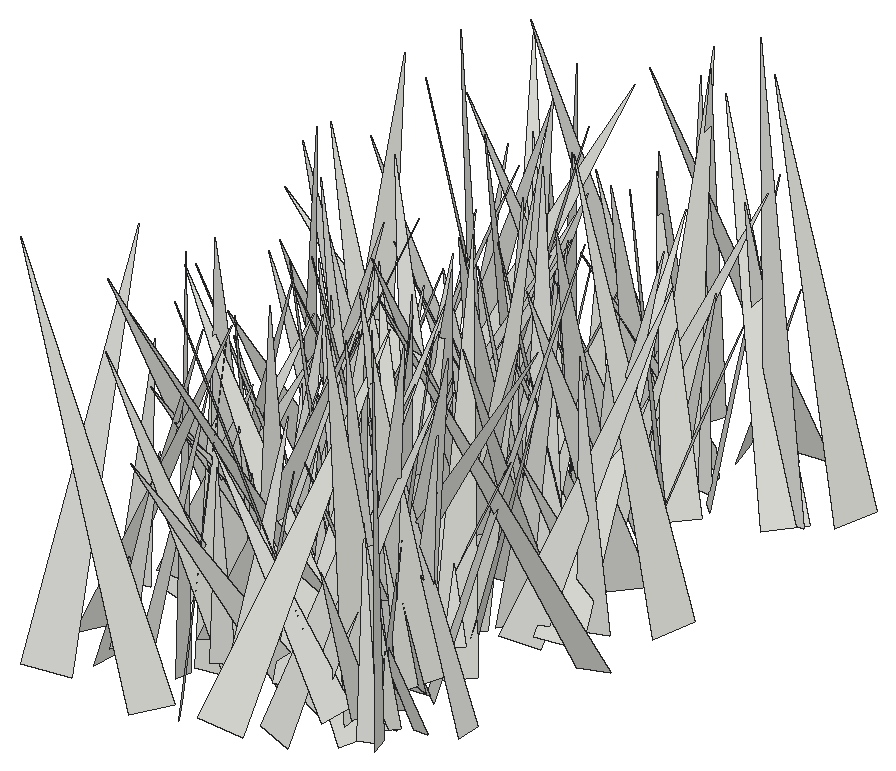
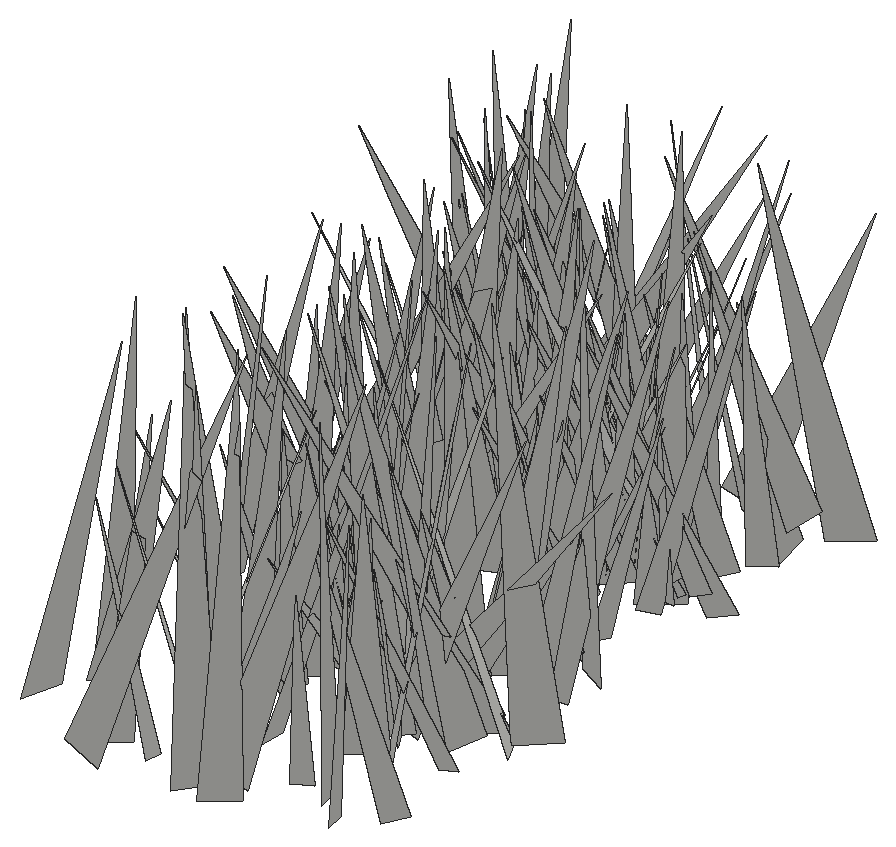
# SketchUp Ruby script. Lengths in inches.
U = 1.inch
M = Sketchup.active_model
def pt(a) = Geom::Point3d.new(a.map { |v| v * U })
def face(e, loops, mat)
  f = e.add_face(loops[0].map { |a| pt(a) })
  loops[1..].each { |l| e.add_face(l.map { |a| pt(a) }).erase! }
  f.material = f.back_material = mat if mat
  f
end
# faces: each face lists its corners as indices into pts; further lists are holes
def faces(e, pts, list, mat = nil) = list.each { |f| face(e, (f[0].is_a?(Array) ? f : [f]).map { |l| l.map { |i| pts[i] } }, mat) }
# xy, xz, yz: faces in a plane at the given z, y or x. An outline is a flat list of corners, or four numbers for a rectangle; further outlines are holes
def ring(l) = l.size == 4 ? [[l[0], l[1]], [l[2], l[1]], [l[2], l[3]], [l[0], l[3]]] : l.each_slice(2).to_a
def flat(e, list, mat, &to3) = list.each { |f| face(e, (f[0].is_a?(Array) ? f : [f]).map { |l| ring(l).map { |u, v| to3.(u, v) } }, mat) }
def xy(e, z, list, mat = nil) = flat(e, list, mat) { |x, y| [x, y, z] }
def xz(e, y, list, mat = nil) = flat(e, list, mat) { |x, z| [x, y, z] }
def yz(e, x, list, mat = nil) = flat(e, list, mat) { |y, z| [x, y, z] }
def lines(e, pts, list) = list.each { |a, b| e.add_line(pt(pts[a]), pt(pts[b])) }
# prism: a flat outline (further loops are holes) pulled along v
def prism(e, loops, v, mat = nil)
  f = face(e, loops, mat); d = Geom::Vector3d.new(v.map { |x| x * U })
  f.pushpull(f.normal.samedirection?(d) ? d.length : -d.length)
end
def box(e, o, s, mat = nil) = prism(e, [[o, [o[0] + s[0], o[1], o[2]], [o[0] + s[0], o[1] + s[1], o[2]], [o[0], o[1] + s[1], o[2]]]], [0, 0, s[2]], mat)
def at(x, y, z, deg = 0) = Geom::Transformation.translation(pt([x, y, z])) * Geom::Transformation.rotation(ORIGIN, Z_AXIS, deg.degrees)
def axes(o, x, y, z) = Geom::Transformation.new([*x, 0, *y, 0, *z, 0, *pt(o).to_a, 1])
def part(name) = M.definitions.add(name)
# library, detail: a bought-in or finely detailed component or shape, given as its bounding box
def library(name, o, s) = part(name).tap { |d| box(d.entities, o, s) }
def detail(e, o, s) = box(e.add_group.entities, o, s)
def put(e, d, t, mat = nil) = e.add_instance(d, t).tap { |i| i.material = mat if mat }
def group(e, t, mat = nil) = e.add_group.tap { |g| g.transformation = t; g.material = mat if mat }.entities
root = M.entities
c1 = part("fur_instance\#9")
p = [[0.8125,0,1.79],[0.67,-0.02,1.48],[0,-0.11,0],[0,0.11,0]]
faces(c1.entities,p,[[0,1,2,3]])
put(root,c1,axes([143.54,146.02,-28.22],[2.44843,-5.51273,0.60157],[-4.8536,-2.44839,-2.68234],[-2.6823,-0.60174,5.40279]))
put(root,c1,axes([140.68,143.08,-28.22],[5.52113,3.74347,2.2115],[4.00437,-5.77059,-0.2291],[-1.6939,-1.44011,6.66663]))
put(root,c1,axes([146.79,144.82,-27.1],[3.04717,-2.22298,0.43436],[-2.028,-3.00193,-1.13631],[-1.00873,-0.67996,3.59662]))
put(root,c1,axes([140.03,142.41,-28.22],[-2.68904,7.46116,1.26428],[7.06219,1.99214,3.26422],[-2.71897,-2.20471,7.22805]))
put(root,c1,axes([143.4375,143.2,-27.1],[4.00682,1.30969,1.18737],[1.29487,-4.17692,0.23764],[-1.20352,-0.13365,4.20874]))
put(root,c1,axes([146.1,144.29,-27.1],[-4.58905,2.11277,0.48874],[2.15665,4.32669,1.54618],[-0.22698,-1.60562,4.80963]))
put(root,c1,axes([138,143.41,-27.1],[3.18405,-1.52738,1.26596],[-1.78098,-3.25535,0.55182],[-0.87386,1.06936,3.48806]))
put(root,c1,axes([143.01,143.0625,-27.1],[-1.4542,4.67664,1.33998],[4.76533,1.65076,-0.58976],[0.97884,-1.08869,4.86188]))
put(root,c1,axes([135.78,142.31,-28.22],[-2.77927,7.20298,1.80131],[7.21654,3.07297,-1.15349],[1.74623,-1.2353,7.63392]))
put(root,c1,axes([145.125,145.05,-27.1],[-5.01465,-5.39389,0.78065],[-5.43536,4.87162,-1.25473],[-0.40033,1.42249,7.25716]))
put(root,c1,axes([143.71,141.3125,-27.1],[-2.62249,6.7547,0.84995],[6.3246,2.75431,-2.37468],[2.5195,0.11678,6.84575]))
put(root,c1,axes([141.24,145.7,-28.22],[-6.5147,0.26004,1.16019],[0.55336,6.38259,1.67669],[1.05235,-1.74639,6.3006]))
put(root,c1,axes([147.95,143.54,-27.1],[-0.46969,3.55211,0.73396],[3.59032,0.35011,0.60316],[-0.51554,-0.79795,3.53189]))
put(root,c1,axes([141.16,144.64,-27.1],[1.90593,-3.10212,1.28599],[-3.27722,-2.04084,-0.06594],[-0.73267,1.05893,3.64024]))
put(root,c1,axes([136.45,143.83,-27.1],[6.61677,-1.08212,0.53072],[-1.15649,-6.53431,1.0953],[-0.3394,1.16883,6.6146]))
put(root,c1,axes([146.45,145.71,-28.22],[4.88048,-6.02987,2.56967],[-6.14977,-5.32095,-0.80587],[-2.26779,1.4525,7.7155]))
put(root,c1,axes([138.1875,144.61,-27.1],[2.95558,3.83246,1.3061],[4.0436,-2.87668,-0.7093],[-0.20723,-1.47175,4.78749]))
put(root,c1,axes([148.43,143.57,-27.1],[-6.12572,-2.31991,2.2614],[-2.97153,5.95041,-1.94497],[1.2907,2.68904,6.25488]))
put(root,c1,axes([146.09,147.31,-28.22],[-2.23996,-8.03771,0.28468],[-7.44594,1.96073,-3.22749],[-3.04036,1.11981,7.69451]))
put(root,c1,axes([136.8125,144.06,-28.22],[6.05583,0.88682,1.38397],[0.67013,-6.15634,1.01257],[-1.50092,0.82941,6.03608]))
put(root,c1,axes([144.86,144.31,-27.1],[1.84734,5.85191,0.92453],[5.8229,-1.61485,-1.41361],[1.09242,-1.28828,5.97153]))
put(root,c1,axes([146.15,146.26,-28.22],[0.04247,-7.07988,2.41623],[-7.48051,-0.06275,-0.05238],[-0.06984,2.41579,7.07981]))
put(root,c1,axes([138.84,147.71,-27.1],[3.08843,-3.08617,0.55459],[-2.71507,-3.02147,-1.69397],[-1.56857,-0.84658,4.0241]))
put(root,c1,axes([140.03,145.85,-27.1],[6.60673,-3.01857,0.44503],[-3.04917,-6.49303,1.22551],[0.11127,1.29906,7.15953]))
put(root,c1,axes([141.49,146.93,-28.22],[6.66168,-2.88093,2.18206],[-2.80757,-7.00677,-0.67958],[-2.27567,0.211,7.22605]))
put(root,c1,axes([147.64,146.68,-28.22],[-2.3451,-4.39084,0.71964],[-4.31416,2.04482,-1.58228],[-1.08875,1.35503,4.71968]))
put(root,c1,axes([146.47,145.2,-28.22],[-4.02573,7.19257,0.41274],[6.48293,3.4104,3.80141],[-3.14246,-2.17854,7.31361]))
put(root,c1,axes([143.54,144.78,-27.1],[-0.09668,3.9627,0.07364],[3.92699,0.08582,0.53775],[-0.5359,-0.08606,3.92724]))
put(root,c1,axes([144.19,143.48,-28.22],[2.76635,7.35948,0.05567],[7.35952,-2.76581,-0.07342],[0.04914,-0.07794,7.86188]))
put(root,c1,axes([144.94,147.53,-28.22],[0.67729,-7.55263,2.0847],[-7.70125,-0.25666,1.57216],[1.44182,2.17688,7.41817]))
put(root,c1,axes([145.24,146.55,-27.1],[-2.81459,-5.30869,2.75415],[-5.79641,3.17103,0.18862],[1.47279,2.33491,6.00571]))
put(root,c1,axes([145.86,148.62,-28.22],[0.26999,-5.16111,0.17986],[-5.16087,-0.27616,-0.17741],[-0.18667,0.17024,5.16512]))
put(root,c1,axes([143.51,145.55,-27.1],[-1.89071,3.52857,0.74513],[3.44423,2.01617,-0.80816],[1.06925,-0.25501,3.92077]))
put(root,c1,axes([146.96,147.55,-27.1],[-6.28621,2.90163,2.83322],[3.4688,6.55463,0.9835],[2.10096,-2.14018,6.85337]))
put(root,c1,axes([135.69,146.93,-27.1],[2.1664,-3.98299,1.68795],[-4.30586,-2.16689,0.41322],[-0.41582,1.68731,4.51516]))
put(root,c1,axes([139.41,144.8,-28.22],[-6.50203,-1.48304,1.94789],[-2.15091,6.10063,-2.53495],[1.1693,2.97539,6.16846]))
put(root,c1,axes([139.86,145.51,-28.22],[0.38602,5.6901,1.15392],[5.67114,-0.61727,1.14668],[-1.24374,-1.04858,5.58671]))
put(root,c1,axes([140.44,147.79,-27.1],[3.55115,-1.15094,1.45453],[-0.93925,-3.82501,-0.73353],[-1.59941,-0.30919,3.66022]))
put(root,c1,axes([139.62,148.21,-28.22],[3.24769,-2.54753,0.32293],[-2.51539,-3.26077,-0.4265],[-0.51676,-0.13836,4.10555]))
put(root,c1,axes([140.58,146.32,-28.22],[-2.71022,2.78687,0.60598],[2.7235,2.77712,-0.59105],[0.8464,-0.01233,3.84222]))
put(root,c1,axes([144.8,147.25,-27.1],[5.13574,3.88277,2.0176],[4.11622,-5.34233,-0.19668],[-1.48436,-1.3806,6.4353]))
put(root,c1,axes([147.13,147.29,-27.1],[-4.91979,-5.33902,1.78444],[-5.59743,4.38767,-2.30455],[-0.5985,2.85253,6.88466]))
put(root,c1,axes([136.66,151.5625,-27.1],[-6.90134,-2.30385,2.57209],[-0.73953,6.60101,3.92832],[3.37291,-3.26662,6.12409]))
put(root,c1,axes([138.62,150.96,-27.1],[-4.47086,-3.62986,0.22446],[-3.11938,4.01034,2.72058],[1.8697,-1.98902,5.07572]))
put(root,c1,axes([141.96,147.96,-27.1],[5.92157,-1.3609,0.111],[-1.36516,-5.91048,0.36315],[-0.02664,0.3788,6.06507]))
put(root,c1,axes([137.95,149.31,-28.22],[5.79688,-5.3049,1.7816],[-5.31494,-6.02201,-0.63769],[-1.75142,0.71643,7.83193]))
put(root,c1,axes([136.31,148.13,-27.1],[2.61538,-3.98544,0.72253],[-3.93735,-2.29982,1.56655],[0.95028,1.43982,4.50221]))
put(root,c1,axes([146.74,145.75,-27.1],[4.8815,3.3845,2.02519],[2.72156,-5.22275,2.16824],[-2.85471,0.80828,5.53015]))
put(root,c1,axes([148.86,147.59,-28.22],[-5.93557,-1.05009,0.32847],[-1.08922,5.86272,-0.94003],[0.15548,0.98355,5.95399]))
put(root,c1,axes([142.375,148.04,-27.1],[-2.65217,1.9255,1.58872],[2.09556,2.97695,-0.10973],[1.35655,-0.83418,3.2756]))
put(root,c1,axes([146,148.55,-27.1],[0.28341,4.29415,2.46111],[4.89058,0.13603,-0.80051],[0.76092,-2.47364,4.22839]))
put(root,c1,axes([139.24,146.98,-28.22],[-2.26569,5.88907,2.62757],[5.5866,3.18358,-2.31806],[3.22106,-1.37923,5.86866]))
put(root,c1,axes([139.6875,147.45,-27.1],[3.18185,3.17768,0.5905],[3.1987,-3.21478,0.06397],[-0.46337,-0.37158,4.49642]))
put(root,c1,axes([144.24,150.39,-27.1],[2.99312,-6.69994,0.30324],[-6.59145,-2.87731,1.48788],[1.23852,0.87852,7.18569]))
put(root,c1,axes([139.23,148.89,-27.1],[4.09073,2.15745,2.5023],[2.51133,-4.61824,-0.12369],[-2.14694,-1.2913,4.62314]))
put(root,c1,axes([143.25,149.18,-28.22],[-5.94217,-4.1756,0.21971],[-4.13273,5.80684,-1.41225],[-0.63601,1.27993,7.12394]))
put(root,c1,axes([144.33,147.29,-28.22],[-6.42625,-2.81034,1.42452],[-3.14557,5.90814,-2.53441],[0.18076,2.90169,6.53999]))
put(root,c1,axes([138.99,151.93,-27.1],[-4.31312,-2.31019,0.44376],[-1.59331,3.55068,2.99849],[1.73068,-2.4885,3.8664]))
put(root,c1,axes([143.48,148.08,-27.1],[6.82569,-2.14516,0.01525],[-2.06759,-6.56497,1.95405],[0.57187,1.86856,6.88284]))
put(root,c1,axes([145.48,146.83,-27.1],[0.70112,8.01126,1.73468],[7.49163,-1.33281,3.12731],[-3.32639,-1.31314,7.4089]))
put(root,c1,axes([137.25,149.21,-27.1],[6.44978,-0.00096,0.92482],[0.04605,-6.50733,-0.32793],[-0.92367,-0.33115,6.44144]))
put(root,c1,axes([144.21,149.79,-27.1],[6.7511,0.38921,2.10678],[0.68602,-6.99103,-0.90679],[-2.02963,-1.06837,6.70124]))
put(root,c1,axes([139.9,148.81,-28.22],[-3.99726,2.72851,1.81883],[2.89094,4.28575,-0.07581],[1.5477,-0.9584,4.83912]))
put(root,c1,axes([140.45,150.31,-27.1],[-2.2334,-3.12116,0.78897],[-3.02774,2.36275,0.77617],[1.09405,0.16724,3.75863]))
put(root,c1,axes([141.28,149.39,-27.1],[-3.78552,-3.06993,0.30173],[-3.01727,3.58565,-1.37288],[-0.64154,1.25071,4.67652]))
put(root,c1,axes([139.8,149.0625,-28.22],[3.39124,-4.48702,2.29298],[-4.9912,-3.37077,0.78574],[-0.69206,2.32297,5.56924]))
put(root,c1,axes([143.09,148.83,-28.22],[-0.70822,-5.57958,3.0516],[-6.3293,0.31925,-0.88519],[-0.61961,3.1164,5.55425]))
put(root,c1,axes([139.74,147.78,-28.22],[7.54644,-1.30772,2.23251],[-1.88035,-7.50036,1.96263],[-1.77721,2.38276,7.40318]))
put(root,c1,axes([144.8,148.04,-28.22],[-5.60196,1.71083,0.59088],[1.59688,5.57635,-1.00614],[0.85208,0.79713,5.77032]))
put(root,c1,axes([142.18,148.34,-28.22],[0.3651,6.79595,1.75212],[7.01816,-0.34958,-0.10649],[0.01583,-1.75528,6.80491]))
put(root,c1,axes([136.06,149.64,-27.1],[1.52671,4.77623,1.67607],[4.63081,-0.61106,-2.47682],[2.04382,-2.18327,4.35989]))
put(root,c1,axes([141.57,149.66,-27.1],[-0.36242,4.3186,2.109],[4.6668,0.82166,-0.88056],[1.14855,-1.97588,4.24338]))
put(root,c1,axes([142.89,149.13,-28.22],[4.31663,-3.25233,1.38409],[-3.53279,-4.03972,1.52536],[-0.11299,2.05661,5.185]))
put(root,c1,axes([139.29,149.96,-28.22],[-4.67685,-1.64881,1.07356],[-1.71505,4.77313,-0.14071],[0.96421,0.49258,4.95698]))
put(root,c1,axes([142.67,149.66,-28.22],[-6.02179,2.8816,2.13168],[3.11245,6.27078,0.31555],[1.77772,-1.21792,6.66828]))
put(root,c1,axes([142.02,150.29,-28.22],[5.34451,-3.5502,0.35957],[-3.55754,-5.25077,1.03462],[0.27778,1.05952,6.33224]))
put(root,c1,axes([145.17,150.3125,-28.22],[3.51099,-0.42801,1.09439],[-0.295,-3.65871,-0.48452],[-1.13748,-0.37227,3.50364]))
put(root,c1,axes([145.62,148.45,-27.1],[-3.34888,5.66427,0.75226],[5.70524,3.26636,0.80369],[-0.31635,-1.05439,6.53093]))
put(root,c1,axes([137.86,149.01,-28.22],[3.23121,-4.00646,1.7311],[-4.24322,-2.37965,2.41277],[1.02152,2.78831,4.54653]))
put(root,c1,axes([138.74,148.24,-27.1],[7.17048,3.0592,0.30714],[3.02615,-7.16002,0.66735],[-0.54355,0.49421,7.76718]))
put(root,c1,axes([136.55,150.6875,-27.1],[-1.07299,-3.39329,1.1863],[-3.30809,1.41653,1.05972],[1.4065,0.74301,3.39746]))
put(root,c1,axes([140.45,149.05,-28.22],[-2.41477,3.3901,0.55663],[3.41153,2.44646,-0.10002],[0.40504,-0.3947,4.161]))
put(root,c1,axes([135.88,148.71,-28.22],[-0.28996,5.60424,1.15409],[5.32871,0.68543,-1.98963],[2.08431,-0.97272,5.24719]))
put(root,c1,axes([144.57,150.93,-27.1],[4.26627,1.55205,0.05399],[1.49304,-4.05567,-1.39111],[0.42732,-1.32496,4.32143]))
put(root,c1,axes([143.57,149.01,-27.1],[-0.37252,4.33667,0.3989],[4.3129,0.31185,0.63743],[-0.60398,-0.44793,4.30572]))
put(root,c1,axes([149.44,153.28,-28.22],[-1.57704,-7.74459,0.50786],[-7.45096,1.36569,-2.31124],[-2.17253,0.93802,7.55804]))
put(root,c1,axes([145.89,149.74,-27.1],[-3.99948,7.12267,1.32626],[7.23474,3.8453,1.16596],[-0.38726,-1.72292,8.0851]))
put(root,c1,axes([144.88,151.57,-27.1],[-3.87014,-4.65436,0.40491],[-4.4497,3.51193,-2.16136],[-1.42379,1.67578,5.65416]))
put(root,c1,axes([146.34,150,-28.22],[-6.2785,3.87073,1.88034],[3.7817,6.55006,-0.85632],[2.05354,-0.22787,7.32591]))
put(root,c1,axes([138.96,150.03,-27.1],[3.99187,0.97882,1.10255],[0.50795,-3.90054,1.62373],[-1.38409,1.39155,3.77579]))
put(root,c1,axes([140.68,152.52,-28.22],[1.01091,-5.94061,2.30759],[-6.04054,-1.63799,-1.57056],[-2.03168,1.91413,5.81775]))
put(root,c1,axes([138.03,152.39,-28.22],[-4.20728,0.83557,0.99678],[1.00115,4.23485,0.67581],[0.83033,-0.87227,4.23588]))
put(root,c1,axes([146.06,151,-28.22],[4.3038,1.80689,1.01933],[1.67441,-4.41138,0.75005],[-1.22483,0.31842,4.60705]))
put(root,c1,axes([146.49,148.62,-28.22],[5.37795,5.75,0.47067],[5.40496,-5.24661,2.33794],[-2.01755,1.27162,7.51791]))
put(root,c1,axes([142.11,149.18,-27.1],[6.07778,0.82962,2.17123],[-0.33597,-5.70106,3.1188],[-2.29992,3.02515,5.28212]))
put(root,c1,axes([139.61,150.81,-28.22],[6.18202,1.83786,0.77531],[1.68935,-6.16651,1.14736],[-1.06062,0.8903,6.34654]))
put(root,c1,axes([145.69,155.46,-28.22],[-0.13701,-6.93499,0.01519],[-6.899,0.13785,0.70555],[0.70571,0.00117,6.90036]))
put(root,c1,axes([136.93,156.4,-28.22],[5.40671,-4.03304,0.21931],[-3.53675,-4.90438,-2.9974],[-1.95061,-2.2864,6.04264]))
put(root,c1,axes([143.93,156.16,-28.22],[1.01288,-8.11783,0.06805],[-8.08119,-1.01477,-0.77093],[-0.77341,-0.02823,8.14437]))
put(root,c1,axes([143.53,153.57,-28.22],[5.79925,-1.98106,0.58125],[-1.98372,-5.82701,-0.06806],[-0.57211,0.1232,6.12791]))
put(root,c1,axes([140.98,151.95,-28.22],[4.10356,-2.98524,2.70877],[-3.77942,-4.1935,1.10399],[-1.40181,2.56732,4.95298]))
put(root,c1,axes([142.13,152.58,-27.1],[-1.06035,5.5551,1.84187],[5.77115,1.30347,-0.60889],[0.97234,-1.67863,5.62252]))
put(root,c1,axes([144.53,152,-27.1],[-2.34195,3.99616,0.3444],[3.99913,2.35703,-0.15486],[0.30802,-0.21845,4.62925]))
put(root,c1,axes([140.72,153.06,-28.22],[-4.50468,1.1443,0.55643],[1.12699,4.53841,-0.20945],[0.5907,0.0676,4.64302]))
put(root,c1,axes([136.6,154.53,-28.22],[4.42565,6.01002,3.52258],[6.87552,-4.43985,-1.06317],[-1.12079,-3.50468,7.38759]))
put(root,c1,axes([138.67,152.47,-27.1],[4.2696,-0.12633,0.87704],[-0.45536,-4.01534,1.6384],[-0.76014,1.6958,3.94476]))
put(root,c1,axes([137.55,153.81,-28.22],[2.6257,3.60497,0.95618],[3.72031,-2.44904,-0.98281],[0.26337,-1.34567,4.35019]))
put(root,c1,axes([139.77,155.17,-28.22],[2.50523,-6.92108,2.84903],[-7.08461,-3.16179,-1.45116],[-2.41383,2.09672,7.21607]))
put(root,c1,axes([144.72,152.66,-28.22],[-6.71814,2.72987,2.53139],[2.23652,7.13443,-1.75826],[2.97626,0.8008,7.03521]))
put(root,c1,axes([139.52,155.93,-28.22],[2.72704,-3.27265,0.76108],[-3.17295,-2.83078,-0.80329],[-1.10537,0.05182,4.1835]))
put(root,c1,axes([139.78,156.94,-28.22],[2.36593,-6.95857,0.28973],[-6.83072,-2.25873,1.53056],[1.359,0.76137,7.18865]))
put(root,c1,axes([147.92,155.16,-28.22],[-1.45922,4.42701,2.15741],[4.90506,1.50733,0.22462],[0.43952,-2.12407,4.65589]))
put(root,c1,axes([146.49,153.2,-28.22],[-3.66435,5.27166,1.90181],[4.6134,4.12758,-2.55233],[3.18179,0.08644,5.89097]))
put(root,c1,axes([146.04,157.25,-28.22],[1.81992,-3.21241,0.00061],[-3.09433,-1.75321,-0.99152],[-0.86298,-0.48823,3.55649]))
put(root,c1,axes([145.55,153.9375,-28.22],[-6.0255,1.4926,2.28597],[0.94971,6.33899,-1.63567],[2.5596,1.16168,5.98825]))
put(root,c1,axes([135.95,158.76,-28.22],[6.25747,-1.85529,1.59771],[-1.00282,-5.94215,-2.97253],[-2.23363,-2.52972,5.81052]))
put(root,c1,axes([147.03,158.13,-28.22],[2.99002,-5.93259,1.12286],[-5.76165,-3.17812,-1.449],[-1.8055,0.31717,6.48354]))
put(root,c1,axes([143.04,158.17,-28.22],[-4.0085,-3.44331,0.94309],[-3.06456,4.04605,1.74695],[1.83147,-0.76613,4.98725]))
put(root,c1,axes([145.98,155.12,-28.22],[-5.43034,-1.89464,0.64767],[-1.9986,5.01546,-2.08529],[-0.12137,2.18018,5.36002]))
put(root,c1,axes([139.04,156.18,-28.22],[-5.93712,3.87569,1.72238],[4.1151,5.9813,0.72589],[1.02637,-1.56207,7.0529]))
put(root,c1,axes([140.62,159.46,-28.22],[6.44625,-4.17663,0.34492],[-3.99481,-6.31514,-1.81045],[-1.26676,-1.33867,7.46462]))
put(root,c1,axes([139.44,157.57,-28.22],[-0.38653,-3.78857,0.47263],[-3.40937,0.1287,-1.7566],[-1.71837,0.59684,3.37891]))
put(root,c1,axes([144.79,156.44,-28.22],[-2.11891,6.73628,2.3501],[7.12334,2.13432,0.30482],[0.39806,-2.33612,7.05509]))
put(root,c1,axes([145.61,157.23,-28.22],[-3.99562,-4.42007,1.47298],[-4.65768,3.83659,-1.12173],[0.11293,1.84803,5.85182]))
put(root,c1,axes([144.3,156.51,-28.22],[-0.05946,3.80591,1.08242],[3.88392,0.26301,-0.71143],[0.75616,-1.05166,3.7393]))
put(root,c1,axes([146.89,155.24,-28.22],[5.43487,-1.88004,3.06705],[-2.9758,-5.47185,1.91904],[-2.02138,3.00059,5.42123]))
put(root,c1,axes([149.84,156.89,-28.22],[-8.02945,1.44749,0.94959],[1.4539,8.08421,-0.0293],[0.93976,-0.13944,8.15883]))
put(root,c1,axes([147.46,153.9375,-28.22],[-4.59589,5.78444,0.11594],[5.4804,4.40003,-2.28044],[1.8543,1.33244,7.02721]))
put(root,c1,axes([145.26,158.89,-28.22],[-0.33962,-4.53633,0.58104],[-4.49375,0.22275,-0.88758],[-0.84975,0.63509,4.46159]))
put(root,c1,axes([144.07,160.23,-28.22],[6.58115,-3.41587,1.26301],[-3.10443,-6.62563,-1.74311],[-1.90417,-1.00387,7.20703]))
put(root,c1,axes([140.33,160.93,-28.22],[-3.25593,-5.45811,0.05054],[-5.36708,3.21208,1.12765],[0.99394,-0.53501,6.25464]))
put(root,c1,axes([137.5,158.04,-28.22],[4.10268,4.53992,0.30052],[4.35228,-3.79801,-2.04106],[1.3262,-1.58032,5.76861]))
put(root,c1,axes([144.11,158.49,-28.22],[-2.65775,-2.55388,1.91088],[-2.80676,3.05414,0.17806],[1.51521,1.17784,3.68161]))
put(root,c1,axes([139.64,159.88,-28.22],[3.7662,-3.06911,1.25827],[-2.92554,-3.97067,-0.92842],[-1.56328,0.03677,4.76883]))
put(root,c1,axes([135.28,158.95,-28.22],[-3.8242,6.03816,3.67075],[6.53219,4.61268,-0.78232],[2.69524,-2.61192,7.10435]))
put(root,c1,axes([139.98,160.03,-28.22],[-5.02457,3.67244,0.21301],[3.24783,4.25941,3.17608],[-1.72736,-2.67378,5.35216]))
put(root,c1,axes([137.86,158.66,-28.22],[3.52755,5.08967,0.59914],[4.90233,-3.13928,-2.19532],[1.49362,-1.71683,5.79042]))
put(root,c1,axes([141.57,158.52,-28.22],[1.56528,5.39191,1.82425],[5.61252,-1.77733,0.43748],[-0.9488,-1.61836,5.59744]))
put(root,c1,axes([147.85,159.26,-28.22],[3.85266,4.81198,3.39076],[5.17881,-4.69725,0.78179],[-2.79863,-2.06788,6.11449]))
put(root,c1,axes([139.95,161.41,-28.22],[-6.05203,-3.65216,2.90127],[-3.20675,6.70926,1.75646],[3.38709,-0.1736,6.84691]))
put(root,c1,axes([144.54,161.65,-28.22],[-3.8372,-2.33717,0.79383],[-2.01321,3.81242,1.493],[1.42812,-0.90538,4.23762]))
put(root,c1,axes([138.53,157.91,-28.22],[-2.17484,4.53028,0.06229],[4.50087,2.16823,-0.54601],[0.51907,0.1805,4.99552]))
put(root,c1,axes([135.65,159.89,-28.22],[5.98281,3.47845,0.55141],[3.51313,-5.81778,-1.41742],[0.2481,-1.50052,6.77381]))
put(root,c1,axes([139.63,159.02,-28.22],[6.78168,2.91502,1.19431],[2.8839,-6.88568,0.43057],[-1.26762,-0.07012,7.36906]))
put(root,c1,axes([141.36,160.01,-28.22],[3.10895,3.01642,1.49943],[3.22004,-3.26039,-0.11754],[-0.98914,-1.13301,4.33019]))
put(root,c1,axes([139.39,160.77,-28.22],[-0.80032,5.57612,2.90873],[5.9333,-0.30294,2.21326],[-2.08561,-3.00158,5.18026]))
put(root,c1,axes([141.76,159.78,-28.22],[3.54809,3.00738,1.07129],[3.07779,-3.64774,0.04651],[-0.84804,-0.65624,4.65093]))
put(root,c1,axes([143.84,160.81,-28.22],[2.86459,-3.18276,1.27512],[-3.34476,-2.95943,0.1272],[-0.754,1.03614,4.28015]))
put(root,c1,axes([143.34,159.0625,-28.22],[-0.67642,4.08917,0.12939],[3.98053,0.62749,0.97839],[-0.94522,-0.2838,4.0276]))
put(root,c1,axes([139.27,160.57,-28.22],[3.65064,-1.60023,0.53489],[-1.66152,-3.63138,0.47591],[-0.29361,0.65299,3.95745]))
put(root,c1,axes([144.61,160.03,-28.22],[0.16923,4.07191,1.2027],[4.12697,0.12503,-1.00402],[0.99752,-1.2081,3.94982]))
put(root,c1,axes([139.76,159.72,-28.22],[3.6249,6.4726,3.15784],[6.5149,-4.45394,1.65071],[-3.06961,-1.8095,7.23254]))
put(root,c1,axes([137.08,160.46,-28.22],[6.77248,-2.83159,1.61361],[-3.13932,-6.6674,1.47599],[-0.87537,2.00399,7.19067]))
put(root,c1,axes([139.32,161.5,-28.22],[5.01911,-5.50348,2.14134],[-5.83765,-5.04831,0.7082],[-0.89193,2.07156,7.41473]))
put(root,c1,axes([142.14,163.97,-28.22],[-7.65526,-2.65251,1.50577],[-2.23878,7.64939,2.09305],[2.07148,-1.53532,7.82675]))
put(root,c1,axes([138.11,163.04,-28.22],[-5.36571,-5.00333,1.81378],[-4.95811,5.63559,0.87824],[1.93398,0.5664,7.28374]))
put(root,c1,axes([136.86,159.24,-28.22],[0.81957,8.13408,0.73803],[7.68253,-0.51597,-2.84467],[2.77248,-0.97476,7.66439]))
put(root,c1,axes([136.96,161.81,-28.22],[2.3418,4.95634,1.60959],[5.19702,-2.35112,-0.32146],[-0.38351,-1.59595,5.4723]))
put(root,c1,axes([143.1,164.2,-28.22],[5.68928,-3.36377,1.44998],[-3.11585,-5.85243,-1.35122],[-1.92583,-0.46842,6.46971]))
put(root,c1,axes([140.12,160.61,-28.22],[3.83996,1.68055,0.1423],[1.49178,-3.54944,1.66307],[-0.78682,1.47206,3.84756]))
put(root,c1,axes([140.16,161.87,-28.22],[-1.05429,4.67357,0.99792],[4.75005,0.91265,0.74413],[-0.52453,-1.12891,4.73287]))
put(root,c1,axes([139.04,161.26,-28.22],[3.31155,2.43431,1.59522],[1.82743,-3.61986,1.73033],[-2.2652,0.63849,3.72802]))
put(root,c1,axes([136.43,162.05,-28.22],[1.36791,4.73736,0.76135],[4.55305,-1.0318,-1.76027],[1.51392,-1.17738,4.60599]))
put(root,c1,axes([144.91,162.22,-28.22],[3.15167,2.15202,0.19961],[2.1362,-3.1554,0.29004],[-0.32814,0.12762,3.80527]))
put(root,c1,axes([144.09,166.32,-28.22],[-4.33714,-4.09832,0.0827],[-3.81397,4.0787,2.10515],[1.50223,-1.4771,5.58349]))
put(root,c1,axes([145.55,162.67,-28.22],[-4.18107,4.06515,1.12452],[4.17237,4.21812,0.26475],[0.61747,-0.97641,5.82552]))
put(root,c1,axes([144.1875,164.07,-28.22],[2.08402,3.38406,1.47593],[3.68931,-1.84524,-0.97848],[0.13865,-1.76538,3.85196]))
put(root,c1,axes([142.77,162.0625,-28.22],[2.76171,5.55128,0.00194],[5.48471,-2.72826,-0.95829],[0.85713,-0.42855,6.1258]))
put(root,c1,axes([139.93,162.88,-28.22],[-1.29816,5.29172,0.79515],[5.27739,1.13069,1.0911],[-0.88529,-1.01932,5.33826]))
put(root,c1,axes([144.24,163.7,-28.22],[-5.26533,5.42334,2.66225],[5.51698,5.75546,-0.81326],[2.46233,-1.29842,7.51498]))
put(root,c1,axes([139.16,162.89,-28.22],[-4.42637,5.44798,0.10976],[5.44745,4.42761,-0.08267],[0.13338,-0.03304,7.019]))
put(root,c1,axes([135.74,165.66,-28.22],[2.085,-4.49657,0.98747],[-4.39792,-1.62495,1.88661],[1.36107,1.63764,4.58334]))
put(root,c1,axes([142.85,165.41,-28.22],[-1.13244,4.66111,1.93868],[4.91983,0.57378,1.4943],[-1.13125,-2.17064,4.55801]))
put(root,c1,axes([140.93,168.16,-28.22],[6.38115,-3.67921,0.2036],[-3.55943,-6.25987,-1.56256],[-0.95316,-1.25481,7.1982]))
put(root,c1,axes([138.33,165.72,-28.22],[-5.78196,-1.74059,3.08913],[-1.82129,6.52793,0.26926],[3.04225,0.59997,6.03227]))
put(root,c1,axes([148.2,164.61,-28.22],[0.66704,7.88186,2.68055],[8.14998,-1.16705,1.40349],[-1.69907,-2.50365,7.78452]))
put(root,c1,axes([144.65,164.5625,-28.22],[1.28068,6.67783,2.12971],[6.86225,-1.63556,1.00185],[-1.42781,-1.87102,6.72532]))
put(root,c1,axes([148.46,164.31,-28.22],[-4.59485,5.55244,0.46156],[5.5505,4.50971,1.00485],[-0.48434,-0.99407,7.1367]))
put(root,c1,axes([141.74,166.78,-28.22],[-0.48012,-7.554,2.16495],[-7.6037,-0.10085,-2.03814],[-1.98335,2.21526,7.28968]))
put(root,c1,axes([145.71,163.83,-28.22],[3.8094,4.08661,1.06154],[3.80016,-3.94157,1.53675],[-1.84012,0.32005,5.37125]))
put(root,c1,axes([139.54,165.71,-28.22],[1.56835,-2.82264,1.69633],[-3.20586,-1.73838,0.07137],[-0.75322,1.52161,3.2283]))
put(root,c1,axes([145.92,167.29,-28.22],[4.56733,-2.95407,1.62637],[-2.80415,-4.84794,-0.93072],[-1.87305,0.05455,5.35918]))
put(root,c1,axes([137.18,166.97,-28.22],[-4.30625,-1.78107,2.16646],[-1.55574,4.81995,0.87021],[2.33354,-0.07334,4.57807]))
put(root,c1,axes([142.1,167.95,-28.22],[7.09602,-3.54407,1.49132],[-3.45875,-7.25092,-0.77408],[-1.67974,-0.04148,7.89397]))
put(root,c1,axes([149.86,166.17,-28.22],[-7.39383,1.79038,1.19471],[1.82356,7.48136,0.07416],[1.14343,-0.35412,7.60715]))
put(root,c1,axes([144.375,167.3,-28.22],[4.32257,0.5968,0.21737],[0.63053,-4.21214,-0.97382],[-0.07654,-0.99484,4.25352]))
put(root,c1,axes([146.32,168.55,-28.22],[-1.86183,-7.54983,1.10161],[-7.50699,1.61006,-1.65309],[-1.3633,1.44488,7.59827]))
